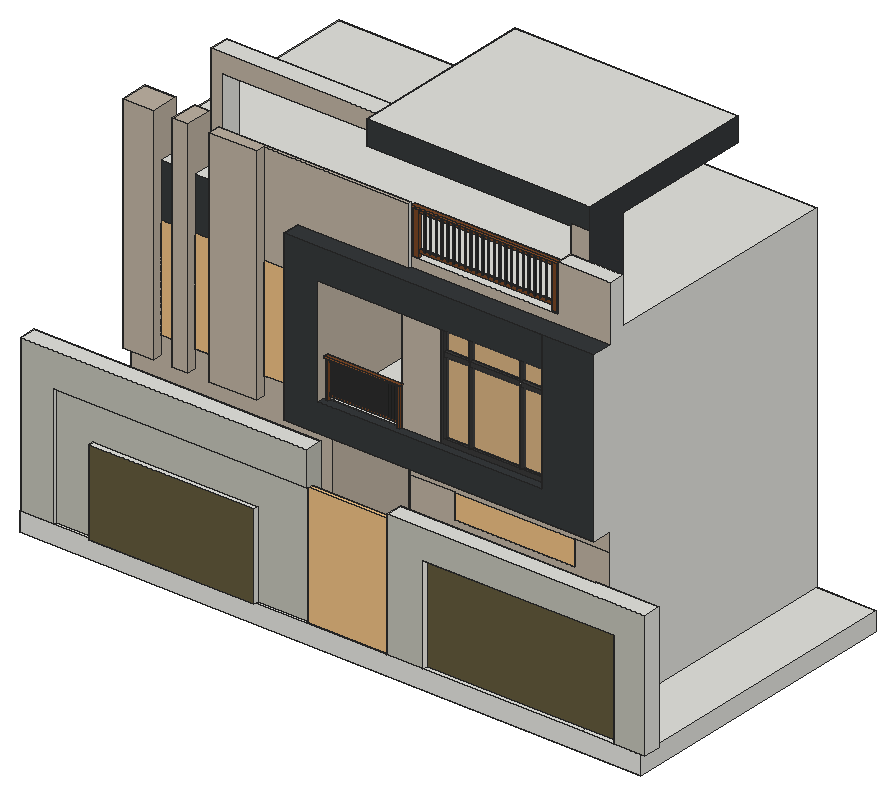
# SketchUp Ruby script. Lengths in inches.
U = 1.inch
M = Sketchup.active_model
def pt(a) = Geom::Point3d.new(a.map { |v| v * U })
def face(e, loops, mat)
  f = e.add_face(loops[0].map { |a| pt(a) })
  loops[1..].each { |l| e.add_face(l.map { |a| pt(a) }).erase! }
  f.material = f.back_material = mat if mat
  f
end
# faces: each face lists its corners as indices into pts; further lists are holes
def faces(e, pts, list, mat = nil) = list.each { |f| face(e, (f[0].is_a?(Array) ? f : [f]).map { |l| l.map { |i| pts[i] } }, mat) }
# xy, xz, yz: faces in a plane at the given z, y or x. An outline is a flat list of corners, or four numbers for a rectangle; further outlines are holes
def ring(l) = l.size == 4 ? [[l[0], l[1]], [l[2], l[1]], [l[2], l[3]], [l[0], l[3]]] : l.each_slice(2).to_a
def flat(e, list, mat, &to3) = list.each { |f| face(e, (f[0].is_a?(Array) ? f : [f]).map { |l| ring(l).map { |u, v| to3.(u, v) } }, mat) }
def xy(e, z, list, mat = nil) = flat(e, list, mat) { |x, y| [x, y, z] }
def xz(e, y, list, mat = nil) = flat(e, list, mat) { |x, z| [x, y, z] }
def yz(e, x, list, mat = nil) = flat(e, list, mat) { |y, z| [x, y, z] }
def lines(e, pts, list) = list.each { |a, b| e.add_line(pt(pts[a]), pt(pts[b])) }
# prism: a flat outline (further loops are holes) pulled along v
def prism(e, loops, v, mat = nil)
  f = face(e, loops, mat); d = Geom::Vector3d.new(v.map { |x| x * U })
  f.pushpull(f.normal.samedirection?(d) ? d.length : -d.length)
end
def box(e, o, s, mat = nil) = prism(e, [[o, [o[0] + s[0], o[1], o[2]], [o[0] + s[0], o[1] + s[1], o[2]], [o[0], o[1] + s[1], o[2]]]], [0, 0, s[2]], mat)
def at(x, y, z, deg = 0) = Geom::Transformation.translation(pt([x, y, z])) * Geom::Transformation.rotation(ORIGIN, Z_AXIS, deg.degrees)
def axes(o, x, y, z) = Geom::Transformation.new([*x, 0, *y, 0, *z, 0, *pt(o).to_a, 1])
def part(name) = M.definitions.add(name)
# library, detail: a bought-in or finely detailed component or shape, given as its bounding box
def library(name, o, s) = part(name).tap { |d| box(d.entities, o, s) }
def detail(e, o, s) = box(e.add_group.entities, o, s)
def put(e, d, t, mat = nil) = e.add_instance(d, t).tap { |i| i.material = mat if mat }
def group(e, t, mat = nil) = e.add_group.tap { |g| g.transformation = t; g.material = mat if mat }.entities
root = M.entities
M.materials.add("0848 AP 9853 Moss Mud-N").color = [98, 89, 60]
M.materials.add("0851 AP 7778 LIMON").color = [192, 192, 181]
M.materials.add("COLOUR").color = [189, 177, 161]
M.materials.add("MADEIRAS PORTAS MOD 4").color = [48, 37, 30]
M.materials.add("Metal_07").color = [114, 116, 119]
M.materials.add("[Color M00]").color = [255, 255, 255]
M.materials.add("[Color_000]1").color = [255, 255, 255]
M.materials.add("[Color_007]").color = [58, 58, 58]
M.materials.add("[Color_D20]").color = [54, 57, 59]
M.materials.add("[Metal Corrugated Shiny]1").color = [192, 192, 192]
M.materials.add("[Metal Seamed]1").color = [37, 38, 36]
M.materials.add("[Steel Brushed Stainless]").color = [183, 187, 190]
M.materials.add("[Translucent Glass Gray]").color = [128, 128, 128]
M.materials["[Translucent Glass Gray]"].alpha = 0.5
M.materials.add("[Translucent_Glass_Gray]1").color = [128, 128, 128]
M.materials["[Translucent_Glass_Gray]1"].alpha = 0.2
M.materials.add("[Wood Veneer 01]").color = [120, 70, 37]
M.materials.add("[Wood_Cherry_Original]2").color = [152, 86, 42]
M.materials.add("aidan_hegarty_redux").color = [127, 127, 127]
M.materials["aidan_hegarty_redux"].alpha = 0
M.materials.add("wood _table").color = [169, 145, 123]
M.materials.add("材料5").color = [245, 242, 234]
c1 = part("Handle mounting plate")
box(c1.entities,[-0.79,0,0],[1.58,2.36,0.2])
c2 = part("Door pull handle")
xy(c2.entities,-28.59,[[0.39,-0.79,0.19,-0.76,0,-0.68,-0.16,-0.56,-0.29,-0.39,-0.37,-0.2,-0.39,0,1.18,0,1.15,-0.2,1.08,-0.39,0.95,-0.56,0.79,-0.68,0.6,-0.76]])
xy(c2.entities,-13.39,[[-0.39,0,1.18,0.79]])
xy(c2.entities,-12.99,[[-0.39,0,1.18,0.79]])
xy(c2.entities,7.09,[[-0.39,0,1.18,0.79]])
xy(c2.entities,7.48,[[-0.39,0,1.18,0.79]])
xy(c2.entities,30.47,[[0.39,-0.79,0.6,-0.76,0.79,-0.68,0.95,-0.56,1.08,-0.39,1.15,-0.2,1.18,0,-0.39,0,-0.37,-0.2,-0.29,-0.39,-0.16,-0.56,0,-0.68,0.19,-0.76]])
xz(c2.entities,0,[[-0.39,-28.59,1.18,-13.39],[-0.39,-12.99,1.18,7.09],[-0.39,7.48,1.18,30.47]])
xz(c2.entities,0.79,[[-0.39,-13.39,1.18,-12.99],[-0.39,7.09,1.18,7.48]])
yz(c2.entities,-0.39,[[0,-13.39,0.79,-12.99],[0,7.09,0.79,7.48]])
yz(c2.entities,1.18,[[0,-13.39,0.79,-12.99],[0,7.09,0.79,7.48]])
p = [[0.19,-0.76,30.47],[0,-0.68,30.47],[0,-0.68,-28.59],[0.19,-0.76,-28.59],[0.39,-0.79,30.47],[0.39,-0.79,-28.59],
  [0.6,-0.76,30.47],[0.6,-0.76,-28.59],[0.79,-0.68,30.47],[0.79,-0.68,-28.59],[-0.16,-0.56,30.47],[-0.16,-0.56,-28.59],
  [0.95,-0.56,30.47],[0.95,-0.56,-28.59],[-0.29,-0.39,30.47],[-0.29,-0.39,-28.59],[1.08,-0.39,30.47],[1.08,-0.39,-28.59],
  [-0.37,-0.2,30.47],[-0.37,-0.2,-28.59],[1.15,-0.2,30.47],[1.15,-0.2,-28.59],[-0.39,0,30.47],[-0.39,0,7.48],
  [-0.39,0,7.09],[-0.39,0,-12.99],[-0.39,0,-13.39],[-0.39,0,-28.59],[1.18,0,30.47],[1.18,0,-28.59],
  [1.18,0,-13.39],[1.18,0,-12.99],[1.18,0,7.09],[1.18,0,7.48]]
faces(c2.entities,p,[[0,1,2,3],[4,0,3,5],[6,4,5,7],[8,6,7,9],[1,10,11,2],[12,8,9,13],[10,14,15,11],[16,12,13,17],
  [14,18,19,15],[20,16,17,21],[18,22,23,24,25,26,27,19],[28,20,21,29,30,31,32,33]])
put(c2.entities,c1,axes([4.72,0.79,-7.35],[1,0,0],[0,0,1],[0,-1,0]))
c3 = part("Door glazing insert")
xy(c3.entities,0,[[0.79,7.09,8.66,18.9]],"aidan_hegarty_redux")
xy(c3.entities,0.39,[[[-0.39,0.58,0.79,0.58,0.79,5.91,8.66,5.91,8.66,1.18,0.79,1.18,0.79,0.58,9.84,0.58,9.84,58.46,-0.39,58.46,-0.39,57.875,8.66,57.875,8.66,53.15,0.79,53.15,0.79,57.875,-0.39,57.875],[0.79,20.08,8.66,38.98],[0.79,40.16,8.66,51.97],[0.79,7.09,8.66,18.9]]])
xy(c3.entities,0.39,[[0.79,1.18,8.66,5.91],[0.79,20.08,8.66,38.98],[0.79,40.16,8.66,51.97],[0.79,53.15,8.66,57.875]],"[Translucent Glass Gray]")
xz(c3.entities,1.18,[[0.79,0,8.66,0.39]])
xz(c3.entities,5.91,[[0.79,0,8.66,0.39]])
xz(c3.entities,7.09,[[0.79,0,8.66,0.39]])
xz(c3.entities,18.9,[[0.79,0,8.66,0.39]])
xz(c3.entities,20.08,[[0.79,0,8.66,0.39]])
xz(c3.entities,38.98,[[0.79,0,8.66,0.39]])
xz(c3.entities,40.16,[[0.79,0,8.66,0.39]])
xz(c3.entities,51.97,[[0.79,0,8.66,0.39]])
xz(c3.entities,53.15,[[0.79,0,8.66,0.39]])
xz(c3.entities,57.875,[[0.79,0,8.66,0.39]])
yz(c3.entities,-0.39,[[0,0,0.06,0.11,0.13,0.21,0.23,0.29,0.33,0.34,0.45,0.38,0.58,0.39,58.46,0.39,58.34,0.38,58.22,0.35,58.11,0.29,58.01,0.21,57.93,0.11,57.875,0],[57.875,0,57.93,0.11,58.01,0.21,58.11,0.29,58.22,0.35,58.34,0.38,58.46,0.39,58.59,0.38,58.71,0.35,58.82,0.29,58.92,0.21,59,0.11,59.06,0]])
yz(c3.entities,0.79,[[1.18,0,5.91,0.39],[7.09,0,18.9,0.39],[20.08,0,38.98,0.39],[40.16,0,51.97,0.39],[53.15,0,57.875,0.39]])
yz(c3.entities,8.66,[[1.18,0,5.91,0.39],[5.91,0,7.09,0.39],[7.09,0,18.9,0.39],[18.9,0,20.08,0.39],[20.08,0,38.98,0.39],
  [38.98,0,40.16,0.39],[40.16,0,51.97,0.39],[51.97,0,53.15,0.39],[53.15,0,57.875,0.39]])
yz(c3.entities,9.84,[[0,0,59.06,0,59,0.11,58.92,0.21,58.82,0.29,58.71,0.35,58.59,0.38,58.46,0.39,0.58,0.39,0.45,0.38,0.33,0.34,0.23,0.29,0.13,0.21,0.06,0.11]])
p = [[-0.39,0.06,0.11],[-0.39,0,0],[0.79,0,0],[9.84,0,0],[9.84,0.06,0.11],[-0.39,59.06,0],
  [-0.39,59,0.11],[9.84,59,0.11],[9.84,59.06,0],[-0.39,0.13,0.21],[9.84,0.13,0.21],[-0.39,58.92,0.21],
  [9.84,58.92,0.21],[-0.39,0.23,0.29],[9.84,0.23,0.29],[-0.39,58.82,0.29],[9.84,58.82,0.29],[-0.39,0.33,0.34],
  [9.84,0.33,0.34],[-0.39,0.45,0.38],[9.84,0.45,0.38],[-0.39,58.71,0.35],[-0.39,58.59,0.38],[9.84,58.59,0.38],
  [9.84,58.71,0.35],[-0.39,0.58,0.39],[9.84,0.58,0.39],[0.79,0.58,0.39],[-0.39,58.46,0.39],[9.84,58.46,0.39]]
faces(c3.entities,p,[[0,1,2,3,4],[5,6,7,8],[9,0,4,10],[6,11,12,7],[13,9,10,14],[11,15,16,12],[17,13,14,18],[19,17,18,20],
  [21,22,23,24],[15,21,24,16],[25,19,20,26,27],[22,28,29,23]])
lines(c3.entities,p,[[27,2]])
c4 = part("dvere")
xy(c4.entities,0,[[0,-0.2,39.37,1.18]],"MADEIRAS PORTAS MOD 4")
xy(c4.entities,3.9375,[[0,-0.2,39.37,0]],"MADEIRAS PORTAS MOD 4")
xy(c4.entities,11.8125,[[14.96,0,24.41,1.18]],"MADEIRAS PORTAS MOD 4")
xy(c4.entities,70.87,[[14.96,0,24.41,1.18]],"MADEIRAS PORTAS MOD 4")
xy(c4.entities,76.77,[[0,-0.2,39.37,0]],"MADEIRAS PORTAS MOD 4")
xy(c4.entities,78.74,[[0,-0.2,39.37,1.18]],"MADEIRAS PORTAS MOD 4")
xz(c4.entities,-0.2,[[0,0,39.37,3.9375],[0,76.77,39.37,78.74]],"MADEIRAS PORTAS MOD 4")
xz(c4.entities,0,[[[0,3.9375,39.37,76.77],[14.96,11.8125,24.41,70.87]]],"MADEIRAS PORTAS MOD 4")
xz(c4.entities,1.18,[[[0,0,39.37,78.74],[14.96,11.8125,24.41,70.87]]],"MADEIRAS PORTAS MOD 4")
yz(c4.entities,0,[[-0.2,0,-0.2,3.9375,0,3.9375,0,76.77,-0.2,76.77,-0.2,78.74,1.18,78.74,1.18,0]],"MADEIRAS PORTAS MOD 4")
yz(c4.entities,14.96,[[0,11.8125,1.18,70.87]],"MADEIRAS PORTAS MOD 4")
yz(c4.entities,24.41,[[0,11.8125,1.18,70.87]],"MADEIRAS PORTAS MOD 4")
yz(c4.entities,39.37,[[-0.2,0,1.18,0,1.18,78.74,-0.2,78.74,-0.2,77.76,0,76.77,0,3.9375,-0.2,3.9375],[-0.2,76.77,0,76.77,-0.2,77.76]],"MADEIRAS PORTAS MOD 4")
p = [[19.69,0,70.87],[19.69,1.18,78.74],[33.46,0,27.01],[33.46,0,25.4375],[24.41,0,69.69],[23.62,0,69.69],
  [23.62,1.19,69.69]]
lines(c4.entities,p,[[0,1],[2,3],[4,5],[5,6]])
put(c4.entities,c2,at(33.86,-0.79,40.4),"Metal_07")
put(c4.entities,c3,axes([24.41,1.19,11.8125],[-1,0,0],[0,0,1],[0,1,0]),"wood _table")
put(c4.entities,c3,axes([14.96,0,11.8125],[1,0,0],[0,0,1],[0,-1,0]),"MADEIRAS PORTAS MOD 4")
c5 = part("Glazed door leaf")
put(c5.entities,c4,at(80.69,2.95,0),"MADEIRAS PORTAS MOD 4")
c6 = part("Glazed entrance door")
put(c6.entities,c5,at(-80.69,-2.76,0),"MADEIRAS PORTAS MOD 4")
c7 = library("window",[0,0,0],[24,5.5,84.25])
c8 = part("Timber plank")
xy(c8.entities,0.42,[[0,-0.52,5.5,50.89]],"[Wood_Cherry_Original]2")
xy(c8.entities,1.92,[[0,-0.52,5.5,50.89]],"[Wood Veneer 01]")
xz(c8.entities,-0.52,[[0,0.42,5.5,1.92]],"[Wood_Cherry_Original]2")
xz(c8.entities,50.89,[[0,0.42,5.5,1.92]],"[Wood_Cherry_Original]2")
yz(c8.entities,0,[[-0.52,0.42,50.89,1.92]],"[Wood_Cherry_Original]2")
yz(c8.entities,5.5,[[-0.52,0.42,50.89,1.92]],"[Wood_Cherry_Original]2")
c9 = part("Group\#1705")
box(c9.entities,[-1.3,-1.0625,0],[3.5,3.5,48],"[Wood Veneer 01]")
c10 = part("Group\#1697")
box(c10.entities,[0,0,0],[79.94,1.5,3.5],"[Wood Veneer 01]")
c11 = part("Group\#2")
xy(c11.entities,0,[[0.09,0,0.125,0.125],[0.125,0,0.16,0.125]],"[Steel Brushed Stainless]")
xy(c11.entities,0.1,[[0.09,0.0625,0.16,0.125]],"[Steel Brushed Stainless]")
xy(c11.entities,0.16,[[0.09,0.0625,0.16,0.125]],"[Steel Brushed Stainless]")
xy(c11.entities,0.25,[[0.09,0,0.125,0.125],[0.125,0,0.16,0.125]],"[Steel Brushed Stainless]")
xz(c11.entities,0,[[0.09,0,0.16,0,0.1875,0.02,0.21,0.04,0.23,0.0625,0.25,0.09,0.25,0.16,0.23,0.1875,0.21,0.21,0.1875,0.23,0.16,0.25,0.09,0.25,0.0625,0.23,0.04,0.21,0.02,0.1875,0,0.16,0,0.09,0.02,0.0625,0.04,0.04,0.0625,0.02]],"[Steel Brushed Stainless]")
xz(c11.entities,0.0625,[[0.09,0.1,0.16,0.16]],"[Steel Brushed Stainless]")
xz(c11.entities,0.125,[[[0.09,0,0.0625,0.02,0.04,0.04,0.02,0.0625,0,0.09,0,0.16,0.02,0.1875,0.04,0.21,0.0625,0.23,0.09,0.25,0.16,0.25,0.1875,0.23,0.21,0.21,0.23,0.1875,0.25,0.16,0.25,0.09,0.23,0.0625,0.21,0.04,0.1875,0.02,0.16,0],[0.09,0.1,0.16,0.16]]],"[Steel Brushed Stainless]")
yz(c11.entities,0,[[0,0.09,0.125,0.125],[0,0.125,0.125,0.16]],"[Steel Brushed Stainless]")
yz(c11.entities,0.09,[[0.0625,0.1,0.125,0.16]],"[Steel Brushed Stainless]")
yz(c11.entities,0.16,[[0.0625,0.1,0.125,0.16]],"[Steel Brushed Stainless]")
yz(c11.entities,0.25,[[0,0.09,0.125,0.125],[0,0.125,0.125,0.16]],"[Steel Brushed Stainless]")
p = [[0.0625,0,0.02],[0.04,0,0.04],[0.04,0.125,0.04],[0.0625,0.125,0.02],[0.02,0,0.0625],[0.02,0.125,0.0625],
  [0.09,0,0],[0.09,0.125,0],[0.23,0,0.0625],[0.21,0,0.04],[0.21,0.125,0.04],[0.23,0.125,0.0625],
  [0.1875,0,0.02],[0.1875,0.125,0.02],[0.16,0,0],[0.16,0.125,0],[0,0,0.09],[0,0.125,0.09],
  [0.25,0,0.09],[0.25,0.125,0.09],[0,0,0.16],[0.02,0,0.1875],[0.02,0.125,0.1875],[0,0.125,0.16],
  [0.04,0,0.21],[0.04,0.125,0.21],[0.0625,0,0.23],[0.0625,0.125,0.23],[0.09,0,0.25],[0.09,0.125,0.25],
  [0.23,0,0.1875],[0.25,0,0.16],[0.25,0.125,0.16],[0.23,0.125,0.1875],[0.16,0,0.25],[0.1875,0,0.23],
  [0.1875,0.125,0.23],[0.16,0.125,0.25],[0.21,0,0.21],[0.21,0.125,0.21]]
faces(c11.entities,p,[[0,1,2,3],[1,4,5,2],[6,0,3,7],[8,9,10,11],[9,12,13,10],[12,14,15,13],[4,16,17,5],[18,8,11,19],
  [20,21,22,23],[21,24,25,22],[24,26,27,25],[26,28,29,27],[30,31,32,33],[34,35,36,37],[35,38,39,36],[38,30,33,39]],"[Steel Brushed Stainless]")
c12 = part("Group\#1858")
box(c12.entities,[0.95,0,12],[0.75,0.5625,32],"[Metal Seamed]1")
c13 = part("Group\#4")
put(c13.entities,c11,at(0.23,0.5625,0.35))
put(c13.entities,c12,at(-0.95,0,-12),"[Color M00]")
put(c13.entities,c11,at(0.23,0.5625,31.54))
put(c13.entities,c11,at(0.23,0.5625,0.79))
put(c13.entities,c11,at(0.23,0.5625,31.1))
c14 = part("Wood+balcony+Railling")
g1 = group(c14.entities,at(0,3.5,0))
put(g1,c8,axes([0,1,40.21],[0,-1,0],[1.90593,0,0],[0,0,1]))
put(g1,c9,axes([2.4375,-2.2,0],[0,1,0],[-1,0,0],[0,0,0.84637]))
put(g1,c10,axes([3.5,-1,37.125],[1.11327,0,0],[0,-1,0],[0,0,1]))
put(g1,c9,axes([94.9375,-2.2,0],[0,1,0],[-1,0,0],[0,0,0.84637]))
put(g1,c10,axes([3.5,-1,4],[1.11327,0,0],[0,-1,0],[0,0,1]))
put(g1,c13,axes([6.93,-2.5,6.38],[1,0,0],[0,-1,0],[0,0,1]))
g2 = group(g1,at(88.12,-2.5,6.38))
put(g2,c12,axes([-0.95,0,-12],[1,0,0],[0,-1,0],[0,0,1]),"[Color M00]")
put(g2,c11,axes([0.29,-0.5625,0.35],[1,0,0],[0,-1,0],[0,0,1]))
put(g2,c11,axes([0.29,-0.5625,31.54],[1,0,0],[0,-1,0],[0,0,1]))
put(g2,c11,axes([0.29,-0.5625,0.79],[1,0,0],[0,-1,0],[0,0,1]))
put(g2,c11,axes([0.29,-0.5625,31.1],[1,0,0],[0,-1,0],[0,0,1]))
put(g1,c13,axes([10.79,-2.5,6.38],[1,0,0],[0,-1,0],[0,0,1]))
put(g1,c13,axes([14.66,-2.5,6.38],[1,0,0],[0,-1,0],[0,0,1]))
put(g1,c13,axes([18.52,-2.5,6.38],[1,0,0],[0,-1,0],[0,0,1]))
put(g1,c13,axes([22.39,-2.5,6.38],[1,0,0],[0,-1,0],[0,0,1]))
put(g1,c13,axes([26.26,-2.5,6.38],[1,0,0],[0,-1,0],[0,0,1]))
put(g1,c13,axes([30.12,-2.5,6.38],[1,0,0],[0,-1,0],[0,0,1]))
put(g1,c13,axes([33.99,-2.5,6.38],[1,0,0],[0,-1,0],[0,0,1]))
put(g1,c13,axes([37.85,-2.5,6.38],[1,0,0],[0,-1,0],[0,0,1]))
put(g1,c13,axes([41.72,-2.5,6.38],[1,0,0],[0,-1,0],[0,0,1]))
put(g1,c13,axes([45.59,-2.5,6.38],[1,0,0],[0,-1,0],[0,0,1]))
put(g1,c13,axes([49.45,-2.5,6.38],[1,0,0],[0,-1,0],[0,0,1]))
put(g1,c13,axes([53.32,-2.5,6.38],[1,0,0],[0,-1,0],[0,0,1]))
put(g1,c13,axes([57.1875,-2.5,6.38],[1,0,0],[0,-1,0],[0,0,1]))
put(g1,c13,axes([61.05,-2.5,6.38],[1,0,0],[0,-1,0],[0,0,1]))
put(g1,c13,axes([64.92,-2.5,6.38],[1,0,0],[0,-1,0],[0,0,1]))
put(g1,c13,axes([68.78,-2.5,6.38],[1,0,0],[0,-1,0],[0,0,1]))
put(g1,c13,axes([72.65,-2.5,6.38],[1,0,0],[0,-1,0],[0,0,1]))
put(g1,c13,axes([76.52,-2.5,6.38],[1,0,0],[0,-1,0],[0,0,1]))
put(g1,c13,axes([80.38,-2.5,6.38],[1,0,0],[0,-1,0],[0,0,1]))
put(g1,c13,axes([84.25,-2.5,6.38],[1,0,0],[0,-1,0],[0,0,1]))
c15 = library("Pleated curtain set",[0,0,0],[14.46,147.43,135.83])
c16 = library("170_fin_black",[-4.89,-2.76,-3.35],[51.16,5.67,71.46])
c17 = part("Plant")
xy(c17.entities,0,[[6.51,0.48,5,0.62,3.57,1.15,2.33,2.03,1.36,3.2,0.73,4.58,0.48,6.08,0.62,7.59,1.15,9.02,2.03,10.26,3.2,11.23,4.58,11.86,6.08,12.11,7.59,11.97,9.02,11.4375,10.26,10.56,11.23,9.39,11.86,8.01,12.11,6.51,11.97,5,11.4375,3.57,10.56,2.33,9.39,1.36,8.01,0.73]],"[Metal Corrugated Shiny]1")
xy(c17.entities,0.86,[[[6.53,0,4.89,0.15,3.35,0.73,2.01,1.68,0.96,2.95,0.27,4.44,0,6.0625,0.15,7.7,0.73,9.24,1.68,10.58,2.95,11.63,4.44,12.32,6.0625,12.59,7.7,12.44,9.24,11.86,10.58,10.91,11.63,9.64,12.32,8.15,12.59,6.53,12.44,4.89,11.86,3.35,10.91,2.01,9.64,0.96,8.15,0.27],[6.51,0.48,8.01,0.73,9.39,1.36,10.56,2.33,11.4375,3.57,11.97,5,12.11,6.51,11.86,8.01,11.23,9.39,10.26,10.56,9.02,11.4375,7.59,11.97,6.08,12.11,4.58,11.86,3.2,11.23,2.03,10.26,1.15,9.02,0.62,7.59,0.48,6.08,0.73,4.58,1.36,3.2,2.33,2.03,3.57,1.15,5,0.62]]],"[Metal Corrugated Shiny]1")
xy(c17.entities,12.8125,[[6.5,0.69,7.94,0.9375,9.28,1.55,10.4,2.48,11.25,3.67,11.76,5.04,11.9,6.5,11.65,7.94,11.04,9.28,10.11,10.4,8.92,11.25,7.55,11.76,6.09,11.9,4.65,11.65,3.31,11.04,2.1875,10.11,1.34,8.92,0.83,7.55,0.69,6.09,0.9375,4.65,1.55,3.31,2.48,2.1875,3.67,1.34,5.04,0.83]])
xy(c17.entities,13.33,[[[6.52,0.3,8.06,0.56,9.48,1.21,10.69,2.21,11.6,3.49,12.15,4.96,12.29,6.52,12.03,8.06,11.38,9.48,10.38,10.69,9.1,11.6,7.63,12.15,6.07,12.29,4.53,12.03,3.11,11.38,1.9,10.38,0.99,9.1,0.44,7.63,0.3,6.07,0.56,4.53,1.21,3.11,2.21,1.9,3.49,0.99,4.96,0.44],[6.5,0.69,5.04,0.83,3.67,1.34,2.48,2.1875,1.55,3.31,0.9375,4.65,0.69,6.09,0.83,7.55,1.34,8.92,2.1875,10.11,3.31,11.04,4.65,11.65,6.09,11.9,7.55,11.76,8.92,11.25,10.11,10.4,11.04,9.28,11.65,7.94,11.9,6.5,11.76,5.04,11.25,3.67,10.4,2.48,9.28,1.55,7.94,0.9375]]],"[Color_000]1")
xy(c17.entities,14.16,[[[6.53,0,8.15,0.27,9.64,0.96,10.91,2.01,11.86,3.35,12.44,4.89,12.59,6.53,12.32,8.15,11.63,9.64,10.58,10.91,9.24,11.86,7.7,12.44,6.0625,12.59,4.44,12.32,2.95,11.63,1.68,10.58,0.73,9.24,0.15,7.7,0,6.0625,0.27,4.44,0.96,2.95,2.01,1.68,3.35,0.73,4.89,0.15],[6.52,0.3,4.96,0.44,3.49,0.99,2.21,1.9,1.21,3.11,0.56,4.53,0.3,6.07,0.44,7.63,0.99,9.1,1.9,10.38,3.11,11.38,4.53,12.03,6.07,12.29,7.63,12.15,9.1,11.6,10.38,10.69,11.38,9.48,12.03,8.06,12.29,6.52,12.15,4.96,11.6,3.49,10.69,2.21,9.48,1.21,8.06,0.56]]],"[Metal Corrugated Shiny]1")
p = [[5,0.62,0],[6.51,0.48,0],[6.51,0.48,0.86],[5,0.62,0.86],[8.01,0.73,0],[8.01,0.73,0.86],
  [3.57,1.15,0],[3.57,1.15,0.86],[9.39,1.36,0],[9.39,1.36,0.86],[2.33,2.03,0],[2.33,2.03,0.86],
  [10.56,2.33,0],[10.56,2.33,0.86],[1.36,3.2,0],[1.36,3.2,0.86],[11.4375,3.57,0],[11.4375,3.57,0.86],
  [0.73,4.58,0],[0.73,4.58,0.86],[11.97,5,0],[11.97,5,0.86],[0.48,6.08,0],[0.48,6.08,0.86],
  [12.11,6.51,0],[12.11,6.51,0.86],[0.62,7.59,0],[0.62,7.59,0.86],[11.86,8.01,0],[11.86,8.01,0.86],
  [1.15,9.02,0],[1.15,9.02,0.86],[11.23,9.39,0],[11.23,9.39,0.86],[2.03,10.26,0],[2.03,10.26,0.86],
  [10.26,10.56,0],[10.26,10.56,0.86],[3.2,11.23,0],[3.2,11.23,0.86],[9.02,11.4375,0],[9.02,11.4375,0.86],
  [4.58,11.86,0],[4.58,11.86,0.86],[7.59,11.97,0],[7.59,11.97,0.86],[6.08,12.11,0],[6.08,12.11,0.86],
  [4.89,0.15,14.16],[4.89,0.15,0.86],[6.53,0,0.86],[6.53,0,14.16],[8.15,0.27,0.86],[8.15,0.27,14.16],
  [3.35,0.73,14.16],[3.35,0.73,0.86],[9.64,0.96,0.86],[9.64,0.96,14.16],[2.01,1.68,14.16],[2.01,1.68,0.86],
  [10.91,2.01,0.86],[10.91,2.01,14.16],[0.96,2.95,14.16],[0.96,2.95,0.86],[11.86,3.35,0.86],[11.86,3.35,14.16],
  [0.27,4.44,14.16],[0.27,4.44,0.86],[12.44,4.89,0.86],[12.44,4.89,14.16],[0,6.0625,14.16],[0,6.0625,0.86],
  [12.59,6.53,0.86],[12.59,6.53,14.16],[0.15,7.7,14.16],[0.15,7.7,0.86],[12.32,8.15,0.86],[12.32,8.15,14.16],
  [0.73,9.24,14.16],[0.73,9.24,0.86],[11.63,9.64,0.86],[11.63,9.64,14.16],[1.68,10.58,14.16],[1.68,10.58,0.86],
  [10.58,10.91,0.86],[10.58,10.91,14.16],[2.95,11.63,14.16],[2.95,11.63,0.86],[9.24,11.86,0.86],[9.24,11.86,14.16],
  [4.44,12.32,14.16],[4.44,12.32,0.86],[7.7,12.44,0.86],[7.7,12.44,14.16],[6.0625,12.59,14.16],[6.0625,12.59,0.86],
  [5.04,0.83,13.33],[6.5,0.69,13.33],[6.5,0.69,12.8125],[5.04,0.83,12.8125],[7.94,0.9375,13.33],[7.94,0.9375,12.8125],
  [3.67,1.34,13.33],[3.67,1.34,12.8125],[9.28,1.55,13.33],[9.28,1.55,12.8125],[2.48,2.1875,13.33],[2.48,2.1875,12.8125],
  [10.4,2.48,13.33],[10.4,2.48,12.8125],[1.55,3.31,13.33],[1.55,3.31,12.8125],[11.25,3.67,13.33],[11.25,3.67,12.8125],
  [0.9375,4.65,13.33],[0.9375,4.65,12.8125],[11.76,5.04,13.33],[11.76,5.04,12.8125],[0.69,6.09,13.33],[0.69,6.09,12.8125],
  [11.9,6.5,13.33],[11.9,6.5,12.8125],[0.83,7.55,13.33],[0.83,7.55,12.8125],[11.65,7.94,13.33],[11.65,7.94,12.8125],
  [1.34,8.92,13.33],[1.34,8.92,12.8125],[11.04,9.28,13.33],[11.04,9.28,12.8125],[2.1875,10.11,13.33],[2.1875,10.11,12.8125],
  [10.11,10.4,13.33],[10.11,10.4,12.8125],[3.31,11.04,13.33],[3.31,11.04,12.8125],[8.92,11.25,13.33],[8.92,11.25,12.8125],
  [4.65,11.65,13.33],[4.65,11.65,12.8125],[7.55,11.76,13.33],[7.55,11.76,12.8125],[6.09,11.9,13.33],[6.09,11.9,12.8125],
  [4.96,0.44,14.16],[6.52,0.3,14.16],[6.52,0.3,13.33],[4.96,0.44,13.33],[8.06,0.56,14.16],[8.06,0.56,13.33],
  [3.49,0.99,14.16],[3.49,0.99,13.33],[9.48,1.21,14.16],[9.48,1.21,13.33],[2.21,1.9,14.16],[2.21,1.9,13.33],
  [10.69,2.21,14.16],[10.69,2.21,13.33],[1.21,3.11,14.16],[1.21,3.11,13.33],[11.6,3.49,14.16],[11.6,3.49,13.33],
  [0.56,4.53,14.16],[0.56,4.53,13.33],[12.15,4.96,14.16],[12.15,4.96,13.33],[0.3,6.07,14.16],[0.3,6.07,13.33],
  [12.29,6.52,14.16],[12.29,6.52,13.33],[0.44,7.63,14.16],[0.44,7.63,13.33],[12.03,8.06,14.16],[12.03,8.06,13.33],
  [0.99,9.1,14.16],[0.99,9.1,13.33],[11.38,9.48,14.16],[11.38,9.48,13.33],[1.9,10.38,14.16],[1.9,10.38,13.33],
  [10.38,10.69,14.16],[10.38,10.69,13.33],[3.11,11.38,14.16],[3.11,11.38,13.33],[9.1,11.6,14.16],[9.1,11.6,13.33],
  [4.53,12.03,14.16],[4.53,12.03,13.33],[7.63,12.15,14.16],[7.63,12.15,13.33],[6.07,12.29,14.16],[6.07,12.29,13.33]]
faces(c17.entities,p,[[0,1,2,3],[1,4,5,2],[6,0,3,7],[4,8,9,5],[10,6,7,11],[8,12,13,9],[14,10,11,15],[12,16,17,13],
  [18,14,15,19],[16,20,21,17],[22,18,19,23],[20,24,25,21],[26,22,23,27],[24,28,29,25],[30,26,27,31],[28,32,33,29],
  [34,30,31,35],[32,36,37,33],[38,34,35,39],[36,40,41,37],[42,38,39,43],[40,44,45,41],[46,42,43,47],[44,46,47,45],
  [48,49,50,51],[51,50,52,53],[54,55,49,48],[53,52,56,57],[58,59,55,54],[57,56,60,61],[62,63,59,58],[61,60,64,65],
  [66,67,63,62],[65,64,68,69],[70,71,67,66],[69,68,72,73],[74,75,71,70],[73,72,76,77],[78,79,75,74],[77,76,80,81],
  [82,83,79,78],[81,80,84,85],[86,87,83,82],[85,84,88,89],[90,91,87,86],[89,88,92,93],[94,95,91,90],[93,92,95,94],
  [144,145,146,147],[145,148,149,146],[150,144,147,151],[148,152,153,149],[154,150,151,155],[152,156,157,153],[158,154,155,159],[156,160,161,157],
  [162,158,159,163],[160,164,165,161],[166,162,163,167],[164,168,169,165],[170,166,167,171],[168,172,173,169],[174,170,171,175],[172,176,177,173],
  [178,174,175,179],[176,180,181,177],[182,178,179,183],[180,184,185,181],[186,182,183,187],[184,188,189,185],[190,186,187,191],[188,190,191,189]],"[Metal Corrugated Shiny]1")
faces(c17.entities,p,[[96,97,98,99],[97,100,101,98],[102,96,99,103],[100,104,105,101],[106,102,103,107],[104,108,109,105],[110,106,107,111],[108,112,113,109],
  [114,110,111,115],[112,116,117,113],[118,114,115,119],[116,120,121,117],[122,118,119,123],[120,124,125,121],[126,122,123,127],[124,128,129,125],
  [130,126,127,131],[128,132,133,129],[134,130,131,135],[132,136,137,133],[138,134,135,139],[136,140,141,137],[142,138,139,143],[140,142,143,141]],"[Color_000]1")
c18 = part("建立群組\#4")
xy(c18.entities,-3.9375,[[[0,0,310.23,191.73],[7.875,7.875,302.36,183.86]],[79.53,7.875,79.53,44.36,81.49,48.29,83.46,44.36,83.46,7.875],[226.77,7.875,226.77,44.36,228.74,48.29,230.7,44.36,230.7,7.875],[7.875,44.36,7.875,52.23,79.53,52.23,81.49,48.29,79.53,44.36],[83.46,44.36,81.49,48.29,83.46,52.23,226.77,52.23,228.74,48.29,226.77,44.36],
  [230.7,44.36,228.74,48.29,230.7,52.23,302.36,52.23,302.36,44.36],[81.49,48.29,79.53,52.23,79.53,183.86,83.46,183.86,83.46,52.23],[228.74,48.29,226.77,52.23,226.77,183.86,230.7,183.86,230.7,52.23]],"[Color_007]")
xy(c18.entities,0,[[83.46,62.6,81.49,66.54,83.46,70.47]])
xy(c18.entities,0,[[7.875,7.875,79.53,44.36],[83.46,7.875,226.77,44.36],[230.7,7.875,302.36,44.36],[83.46,44.36,226.77,52.23],[7.875,52.23,79.53,183.86],
  [83.46,52.23,226.77,183.86],[230.7,52.23,302.36,183.86]],"[Translucent_Glass_Gray]1")
xy(c18.entities,3.9375,[[[0,0,310.23,191.73],[7.875,7.875,302.36,183.86]],[79.53,7.875,83.46,7.875,83.46,44.36,81.49,48.29,79.53,44.36],[226.77,7.875,230.7,7.875,230.7,44.36,228.74,48.29,226.77,44.36],[7.875,44.36,79.53,44.36,81.49,48.29,79.53,52.23,7.875,52.23],[83.46,44.36,226.77,44.36,228.74,48.29,226.77,52.23,83.46,52.23,81.49,48.29],
  [230.7,44.36,302.36,44.36,302.36,52.23,230.7,52.23,228.74,48.29],[81.49,48.29,83.46,52.23,83.46,183.86,79.53,183.86,79.53,52.23],[228.74,48.29,230.7,52.23,230.7,183.86,226.77,183.86,226.77,52.23]],"[Color_007]")
xz(c18.entities,0,[[0,-3.9375,310.23,3.9375]],"[Color_007]")
xz(c18.entities,7.875,[[79.53,-3.9375,83.46,3.9375],[226.77,-3.9375,230.7,3.9375]])
xz(c18.entities,7.875,[[7.875,-3.9375,79.53,0],[83.46,-3.9375,226.77,0],[230.7,-3.9375,302.36,0],[7.875,0,79.53,3.9375],[83.46,0,226.77,3.9375],
  [230.7,0,302.36,3.9375]],"[Color_007]")
xz(c18.entities,44.36,[[7.875,-3.9375,79.53,0],[83.46,-3.9375,226.77,0],[230.7,-3.9375,302.36,0],[7.875,0,79.53,3.9375],[83.46,0,226.77,3.9375],
  [230.7,0,302.36,3.9375]],"[Color_007]")
xz(c18.entities,52.23,[[7.875,-3.9375,79.53,0],[83.46,-3.9375,226.77,0],[230.7,-3.9375,302.36,0],[7.875,0,79.53,3.9375],[83.46,0,226.77,3.9375],
  [230.7,0,302.36,3.9375]],"[Color_007]")
xz(c18.entities,183.86,[[79.53,-3.9375,83.46,3.9375],[226.77,-3.9375,230.7,3.9375]])
xz(c18.entities,183.86,[[7.875,-3.9375,79.53,0],[83.46,-3.9375,226.77,0],[230.7,-3.9375,302.36,0],[7.875,0,79.53,3.9375],[83.46,0,226.77,3.9375],
  [230.7,0,302.36,3.9375]],"[Color_007]")
xz(c18.entities,191.73,[[0,-3.9375,310.23,3.9375]],"[Color_007]")
yz(c18.entities,0,[[0,-3.9375,191.73,3.9375]],"[Color_007]")
yz(c18.entities,7.875,[[44.36,-3.9375,52.23,3.9375]])
yz(c18.entities,7.875,[[7.875,-3.9375,44.36,0],[52.23,-3.9375,183.86,0],[7.875,0,44.36,3.9375],[52.23,0,183.86,3.9375]],"[Color_007]")
yz(c18.entities,79.53,[[7.875,-3.9375,44.36,0],[52.23,-3.9375,183.86,0],[7.875,0,44.36,3.9375],[52.23,0,183.86,3.9375]],"[Color_007]")
yz(c18.entities,83.46,[[7.875,-3.9375,44.36,0],[52.23,-3.9375,183.86,0],[7.875,0,44.36,3.9375],[52.23,0,183.86,3.9375]],"[Color_007]")
yz(c18.entities,226.77,[[7.875,-3.9375,44.36,0],[52.23,-3.9375,183.86,0],[7.875,0,44.36,3.9375],[52.23,0,183.86,3.9375]],"[Color_007]")
yz(c18.entities,230.7,[[7.875,-3.9375,44.36,0],[52.23,-3.9375,183.86,0],[7.875,0,44.36,3.9375],[52.23,0,183.86,3.9375]],"[Color_007]")
yz(c18.entities,302.36,[[44.36,-3.9375,52.23,3.9375]])
yz(c18.entities,302.36,[[7.875,-3.9375,44.36,0],[52.23,-3.9375,183.86,0],[7.875,0,44.36,3.9375],[52.23,0,183.86,3.9375]],"[Color_007]")
yz(c18.entities,310.23,[[0,-3.9375,191.73,3.9375]],"[Color_007]")
p = [[81.49,48.29,3.9375],[83.46,52.23,3.9375],[83.46,52.23,0],[83.46,52.23,-3.9375],[81.49,48.29,-3.9375],[79.53,44.36,-3.9375],
  [79.53,44.36,0],[79.53,44.36,3.9375],[83.46,44.36,3.9375],[79.53,52.23,3.9375],[79.53,52.23,0],[79.53,52.23,-3.9375],
  [83.46,44.36,-3.9375],[83.46,44.36,0],[228.74,48.29,3.9375],[230.7,52.23,3.9375],[230.7,52.23,0],[230.7,52.23,-3.9375],
  [228.74,48.29,-3.9375],[226.77,44.36,-3.9375],[226.77,44.36,0],[226.77,44.36,3.9375],[230.7,44.36,3.9375],[226.77,52.23,3.9375],
  [226.77,52.23,0],[226.77,52.23,-3.9375],[230.7,44.36,-3.9375],[230.7,44.36,0]]
faces(c18.entities,p,[[0,1,2,3,4,5,6,7],[8,0,9,10,11,4,12,13],[14,15,16,17,18,19,20,21],[22,14,23,24,25,18,26,27]])
xy(root,0,[[89.42,0,89.42,6.375,42.29,6.375,42.29,3.0625,0,3.0625,0,24.625,363.22,24.625,363.22,6.375,298.92,6.375,298.92,0],[465.4,2,465.4,23.5,712.6875,23.5,712.6875,24.625,792.9375,24.625,792.9375,2,753.2,2,753.2,8.8125,511.32,8.8125,511.32,2],[106.375,44.25,106.375,374.5625,712.6875,374.5625,712.6875,46.25,459.71,46.25,459.71,162.625,363.22,162.625,363.22,44.25]])
xy(root,107.875,[[89.42,0,298.92,6.375]])
xy(root,123.4375,[[511.32,2,753.2,8.8125]])
xy(root,152.24,[[516.08,46.25,667.96,60.875]])
xy(root,153.22,[[42.29,3.0625,363.22,6.375]])
xy(root,159.625,[[465.4,2,792.9375,2,792.9375,24.625,712.6875,24.625,712.6875,23.5,465.4,23.5]])
xy(root,183.52,[[516.08,46.25,667.96,60.875]])
xy(root,196.75,[[0,3.0625,363.22,24.625]])
xy(root,207.0625,[[318.89,21.625,318.89,44.25,363.22,44.25,363.22,162.625,459.71,162.625,459.71,46.25,712.6875,46.25,712.6875,21.625]],"[Color_D20]")
xy(root,209.64,[[106.375,32.0625,145.29,44.25],[169.24,32.0625,188.58,44.25],[215.28,32.0625,276.14,44.25]])
xy(root,232.43,[[145.29,44.25,169.24,57],[188.58,44.25,215.28,57],[276.14,44.25,301.48,57]])
xy(root,234.07,[[362.16,32.8125,459.71,185.625]])
xy(root,242.89,[[509.67,32.8125,645.87,220.5625]])
xy(root,242.89,[[362.16,21.625,645.87,32.8125]],"[Color_D20]")
xy(root,363.53,[[145.29,44.25,169.24,57],[188.58,44.25,215.28,57],[276.14,44.25,301.48,57]])
xy(root,379.5625,[[509.67,32.8125,645.87,220.5625]])
xy(root,379.5625,[[362.16,21.625,645.87,32.8125]],"[Color_D20]")
xy(root,384.375,[[362.16,32.8125,459.71,185.625]],"COLOUR")
xy(root,418.875,[[318.89,21.625,712.6875,21.625,712.6875,47.75,459.71,47.75,459.71,44.25,318.89,44.25]],"[Color_D20]")
xy(root,431.25,[[145.29,44.25,169.24,44.25,169.24,88.59,173.24,88.59,173.24,113.44,188.39,113.44,188.39,88.59,186.58,88.59,186.58,67.25,188.58,67.25,188.58,44.25,215.28,44.25,215.28,47.75,645.87,47.75,645.87,120.5625,670.1,120.5625,670.1,67.8125,712.6875,67.8125,712.6875,374.5625,106.375,374.5625,106.375,67.25,145.29,67.25],[169.24,44.25,188.58,67.25],[169.24,67.25,186.58,88.59],[645.87,67.8125,670.1,120.5625]])
xy(root,489.625,[[645.87,47.75,712.6875,67.8125]])
xy(root,492.375,[[106.375,32.0625,145.29,67.25],[169.24,32.0625,188.58,67.25],[215.28,32.0625,276.14,32.0625,276.14,44.25,459.71,44.25,459.71,47.75,215.28,47.75]],"COLOUR")
xy(root,521.52,[[386.96,67.8125,386.96,303.09,670.1,303.09,670.1,120.5625,645.87,120.5625,645.87,67.8125]],"[Color_D20]")
xy(root,524.89,[[188.39,88.59,386.96,113.44]])
xy(root,548.4375,[[173.24,88.59,386.96,113.44]])
xy(root,552.1875,[[386.96,67.8125,670.1,303.09]])
xz(root,0,[[89.42,0,298.92,107.875]],"0848 AP 9853 Moss Mud-N")
xz(root,2,[[465.4,0,511.32,0,511.32,123.4375,753.2,123.4375,753.2,0,792.9375,0,792.9375,159.625,465.4,159.625]],"0851 AP 7778 LIMON")
xz(root,3.0625,[[0,0,42.29,0,42.29,153.22,363.22,153.22,363.22,196.75,0,196.75]],"0851 AP 7778 LIMON")
xz(root,6.375,[[42.29,0,89.42,0,89.42,107.875,298.92,107.875,298.92,0,363.22,0,363.22,153.22,42.29,153.22]],"0851 AP 7778 LIMON")
xz(root,8.8125,[[511.32,0,753.2,123.4375]],"0848 AP 9853 Moss Mud-N")
xz(root,21.625,[[318.89,207.0625,712.6875,207.0625,712.6875,418.875,645.87,418.875,645.87,242.89,362.16,242.89,362.16,379.5625,645.87,379.5625,645.87,418.875,318.89,418.875]],"[Color_D20]")
xz(root,23.5,[[465.4,0,712.6875,159.625]])
xz(root,24.625,[[0,0,363.22,196.75],[712.6875,0,792.9375,159.625]])
xz(root,32.0625,[[106.375,209.64,145.29,492.375],[169.24,209.64,188.58,492.375],[215.28,209.64,276.14,492.375]],"COLOUR")
xz(root,32.8125,[[362.16,234.07,459.71,242.89],[362.16,379.5625,459.71,384.375]])
xz(root,32.8125,[[459.71,242.89,509.67,379.5625]],"COLOUR")
xz(root,44.25,[[169.24,209.64,188.58,232.43],[215.28,209.64,276.14,232.43],[169.24,232.43,188.58,363.53],[215.28,232.43,276.14,363.53],[169.24,363.53,188.58,431.25],
  [215.28,363.53,276.14,431.25]])
xz(root,44.25,[[106.375,0,363.22,0,363.22,207.0625,318.89,207.0625,318.89,418.875,459.71,418.875,459.71,492.375,276.14,492.375,276.14,363.53,301.48,363.53,301.48,232.43,276.14,232.43,276.14,209.64,215.28,209.64,215.28,232.43,188.58,232.43,188.58,209.64,169.24,209.64,169.24,232.43,145.29,232.43,145.29,209.64,106.375,209.64]],"COLOUR")
xz(root,44.25,[[145.29,363.53,169.24,431.25],[188.58,363.53,215.28,431.25]],"[Color_D20]")
xz(root,46.25,[[459.71,0,712.6875,0,712.6875,183.52,667.96,183.52,667.96,152.24,516.08,152.24,516.08,183.52,459.71,183.52],[459.71,183.52,712.6875,207.0625]],"COLOUR")
xz(root,47.75,[[215.28,431.25,459.71,492.375]])
xz(root,47.75,[[459.71,418.875,712.6875,418.875,712.6875,489.625,645.87,489.625,645.87,431.25,459.71,431.25]],"COLOUR")
xz(root,57,[[145.29,232.43,169.24,363.53],[188.58,232.43,215.28,363.53],[276.14,232.43,301.48,363.53]])
xz(root,60.875,[[516.08,152.24,667.96,183.52]])
xz(root,67.25,[[106.375,431.25,145.29,492.375],[169.24,431.25,188.58,492.375]])
xz(root,67.8125,[[645.87,431.25,670.1,489.625],[670.1,431.25,712.6875,489.625]])
xz(root,67.8125,[[645.87,489.625,670.1,524.89]],"COLOUR")
xz(root,67.8125,[[386.96,521.52,645.87,521.52,645.87,524.89,670.1,524.89,670.1,552.1875,386.96,552.1875]],"[Color_D20]")
xz(root,88.59,[[173.24,431.25,188.39,431.25,188.39,524.89,386.96,524.89,386.96,548.4375,173.24,548.4375]],"COLOUR")
xz(root,113.44,[[173.24,431.25,173.24,548.4375,386.96,548.4375,386.96,524.89,188.39,524.89,188.39,431.25]])
xz(root,120.5625,[[645.87,431.25,670.1,521.52]])
xz(root,162.625,[[363.22,0,459.71,207.0625]],"COLOUR")
xz(root,185.625,[[362.16,234.07,459.71,384.375]],"COLOUR")
xz(root,220.5625,[[509.67,242.89,645.87,379.5625]])
xz(root,303.09,[[386.96,521.52,670.1,552.1875]])
xz(root,374.5625,[[106.375,0,712.6875,431.25]])
yz(root,0,[[3.0625,0,24.625,196.75]],"材料5")
yz(root,42.29,[[3.0625,0,6.375,153.22]])
yz(root,89.42,[[0,0,6.375,107.875]])
yz(root,106.375,[[44.25,0,44.25,209.64,32.0625,209.64,32.0625,492.375,67.25,492.375,67.25,431.25,374.5625,431.25,374.5625,0]],"0851 AP 7778 LIMON")
yz(root,145.29,[[32.0625,209.64,44.25,209.64,44.25,232.43,57,232.43,57,363.53,44.25,363.53,44.25,431.25,67.25,431.25,67.25,492.375,32.0625,492.375]],"COLOUR")
yz(root,169.24,[[44.25,232.43,57,363.53]])
yz(root,169.24,[[32.0625,209.64,32.0625,492.375,67.25,492.375,67.25,431.25,44.25,431.25,44.25,209.64]],"COLOUR")
yz(root,173.24,[[88.59,431.25,113.44,548.4375]],"COLOUR")
yz(root,188.39,[[88.59,431.25,113.44,524.89]])
yz(root,188.58,[[44.25,232.43,57,363.53]])
yz(root,188.58,[[32.0625,209.64,44.25,209.64,44.25,431.25,67.25,431.25,67.25,492.375,32.0625,492.375]],"COLOUR")
yz(root,215.28,[[44.25,232.43,57,363.53]])
yz(root,215.28,[[32.0625,209.64,32.0625,492.375,47.75,492.375,47.75,431.25,44.25,431.25,44.25,209.64]],"COLOUR")
yz(root,276.14,[[44.25,232.43,57,363.53]])
yz(root,276.14,[[32.0625,209.64,44.25,492.375]],"COLOUR")
yz(root,298.92,[[0,0,6.375,107.875]])
yz(root,301.48,[[44.25,232.43,57,363.53]])
yz(root,318.89,[[21.625,207.0625,44.25,418.875]],"[Color_D20]")
yz(root,362.16,[[32.8125,234.07,185.625,234.07,185.625,384.375,32.8125,384.375,32.8125,379.5625,21.625,379.5625,21.625,242.89,32.8125,242.89]],"COLOUR")
yz(root,363.22,[[6.375,0,24.625,0,24.625,196.75,3.0625,196.75,3.0625,153.22,6.375,153.22]],"0851 AP 7778 LIMON")
yz(root,363.22,[[44.25,0,162.625,207.0625]],"COLOUR")
yz(root,386.96,[[88.59,524.89,113.44,548.4375]])
yz(root,386.96,[[88.59,521.52,113.44,524.89],[88.59,548.4375,113.44,552.1875]],"COLOUR")
yz(root,386.96,[[67.8125,521.52,88.59,552.1875],[113.44,521.52,303.09,552.1875]],"[Color_D20]")
yz(root,459.71,[[44.25,418.875,47.75,492.375]])
yz(root,459.71,[[46.25,0,162.625,207.0625],[32.8125,234.07,185.625,384.375]],"COLOUR")
yz(root,465.4,[[2,0,23.5,159.625]],"材料5")
yz(root,509.67,[[32.8125,242.89,220.5625,379.5625]])
yz(root,511.32,[[2,0,8.8125,123.4375]],"材料5")
yz(root,516.08,[[46.25,152.24,60.875,183.52]])
yz(root,645.87,[[21.625,379.5625,24.625,379.5625,21.625,418.875]])
yz(root,645.87,[[47.75,431.25,67.8125,489.625],[67.8125,431.25,120.5625,521.52]],"COLOUR")
yz(root,645.87,[[21.625,242.89,220.5625,379.5625]],"[Color_D20]")
yz(root,667.96,[[46.25,152.24,60.875,183.52]])
yz(root,670.1,[[67.8125,431.25,120.5625,431.25,120.5625,521.52,303.09,521.52,303.09,552.1875,67.8125,552.1875]],"[Color_D20]")
yz(root,712.6875,[[46.25,0,374.5625,0,374.5625,431.25,67.8125,431.25,67.8125,489.625,47.75,489.625,47.75,418.875,21.625,418.875,21.625,207.0625,46.25,207.0625],[23.5,0,24.625,159.625]])
yz(root,753.2,[[2,0,8.8125,123.4375]])
yz(root,792.9375,[[2,0,24.625,159.625]])
p = [[1656.48,-1123.35,159.23],[1655.48,-1123.35,159.23],[1655.48,-1122.35,159.23]]
lines(root,p,[[0,1],[1,2],[2,0]])
put(root,c6,axes([381.04,184.25,234.07],[1.5,0,0],[0,1,0],[0,0,1.41]))
put(root,c6,axes([369.92,161.25,0],[1.914,0,0],[0,1,0],[0,0,1.9599]))
put(root,c7,axes([276.14,44.25,232.43],[1.05608,0,0],[0,1,0],[0,0,1.55605]))
put(root,c7,axes([188.58,44.25,232.43],[1.11241,0,0],[0,1,0],[0,0,1.55605]))
put(root,c7,axes([145.29,44.25,232.43],[0.99765,0,0],[0,1,0],[0,0,1.55605]))
put(root,c7,axes([516.08,51.75,152.24],[0,0,1.30367],[0,-1,0],[1.80263,0,0]))
put(root,c14,axes([365.63,29.3125,242.89],[0.98,0,0],[0,1,0],[0,0,1.18]))
put(root,c15,axes([654.48,38.6,244.94],[0,0.88,0],[-1,0,0],[0,0,1]))
put(root,c15,axes([314.7,50.02,232.76],[0,0.88,0],[-1.24,0,0],[0,0,1]))
put(root,c16,axes([372.8,7.6,3.99],[2,0,0],[0,1,0],[0,0,2.1911]))
put(root,c17,at(440.61,167.29,234.07))
put(root,c14,axes([461.61,48.75,431.25],[1.89953,0,0],[0,1,0],[0,0,1.3806]))
g3 = group(root,at(106.375,374.5625,-23.8125))
prism(g3,[[[-106.375,0,23.8125],[606.3125,0,23.8125],[681.1875,0,23.8125],[681.1875,0,0],[-106.375,0,0]]],[0,-372.5625,0])
put(root,c18,axes([509.67,36.75,379.5625],[0.43902,0,0],[0,0,-0.71284],[0,1,0]))
